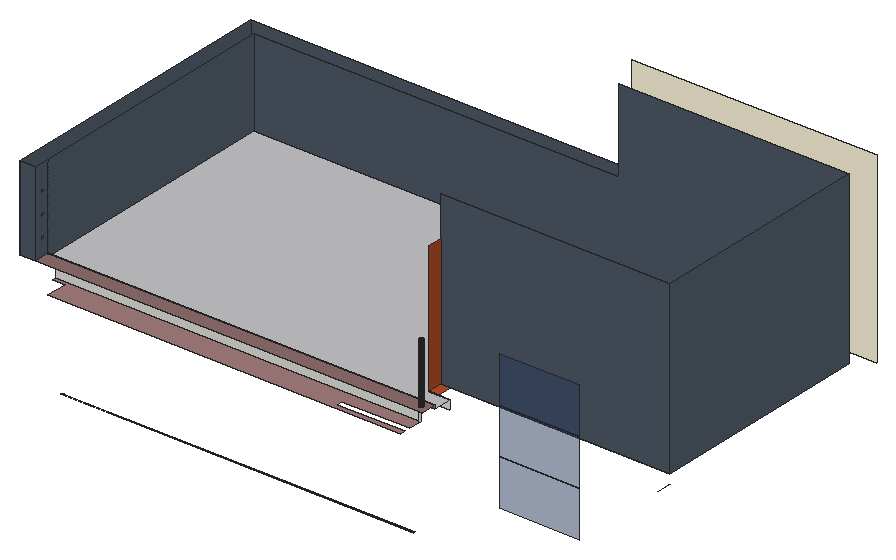
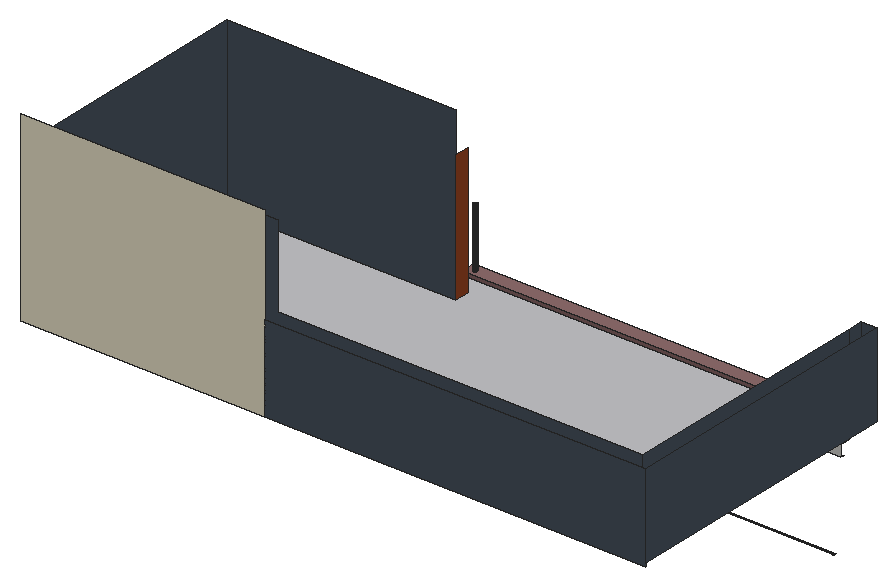
# SketchUp Ruby script. Lengths in inches.
U = 1.inch
M = Sketchup.active_model
def pt(a) = Geom::Point3d.new(a.map { |v| v * U })
def face(e, loops, mat)
  f = e.add_face(loops[0].map { |a| pt(a) })
  loops[1..].each { |l| e.add_face(l.map { |a| pt(a) }).erase! }
  f.material = f.back_material = mat if mat
  f
end
# faces: each face lists its corners as indices into pts; further lists are holes
def faces(e, pts, list, mat = nil) = list.each { |f| face(e, (f[0].is_a?(Array) ? f : [f]).map { |l| l.map { |i| pts[i] } }, mat) }
# xy, xz, yz: faces in a plane at the given z, y or x. An outline is a flat list of corners, or four numbers for a rectangle; further outlines are holes
def ring(l) = l.size == 4 ? [[l[0], l[1]], [l[2], l[1]], [l[2], l[3]], [l[0], l[3]]] : l.each_slice(2).to_a
def flat(e, list, mat, &to3) = list.each { |f| face(e, (f[0].is_a?(Array) ? f : [f]).map { |l| ring(l).map { |u, v| to3.(u, v) } }, mat) }
def xy(e, z, list, mat = nil) = flat(e, list, mat) { |x, y| [x, y, z] }
def xz(e, y, list, mat = nil) = flat(e, list, mat) { |x, z| [x, y, z] }
def yz(e, x, list, mat = nil) = flat(e, list, mat) { |y, z| [x, y, z] }
def lines(e, pts, list) = list.each { |a, b| e.add_line(pt(pts[a]), pt(pts[b])) }
# prism: a flat outline (further loops are holes) pulled along v
def prism(e, loops, v, mat = nil)
  f = face(e, loops, mat); d = Geom::Vector3d.new(v.map { |x| x * U })
  f.pushpull(f.normal.samedirection?(d) ? d.length : -d.length)
end
def box(e, o, s, mat = nil) = prism(e, [[o, [o[0] + s[0], o[1], o[2]], [o[0] + s[0], o[1] + s[1], o[2]], [o[0], o[1] + s[1], o[2]]]], [0, 0, s[2]], mat)
def at(x, y, z, deg = 0) = Geom::Transformation.translation(pt([x, y, z])) * Geom::Transformation.rotation(ORIGIN, Z_AXIS, deg.degrees)
def axes(o, x, y, z) = Geom::Transformation.new([*x, 0, *y, 0, *z, 0, *pt(o).to_a, 1])
def part(name) = M.definitions.add(name)
# library, detail: a bought-in or finely detailed component or shape, given as its bounding box
def library(name, o, s) = part(name).tap { |d| box(d.entities, o, s) }
def detail(e, o, s) = box(e.add_group.entities, o, s)
def put(e, d, t, mat = nil) = e.add_instance(d, t).tap { |i| i.material = mat if mat }
def group(e, t, mat = nil) = e.add_group.tap { |g| g.transformation = t; g.material = mat if mat }.entities
root = M.entities
M.materials.add("[0033_NavajoWhite]").color = [221, 193, 150]
M.materials.add("[0051_Cornsilk]").color = [255, 248, 220]
M.materials.add("[0111_SlateGray]").color = [79, 90, 102]
M.materials.add("[0119_RosyBrown]").color = [142, 108, 108]
M.materials.add("[0119_RosyBrown]1").color = [163, 124, 124]
M.materials.add("[0136_Charcoal]").color = [35, 35, 35]
M.materials.add("[Beadboard]").color = [181, 77, 41]
M.materials.add("[Cladding Siding Tan]").color = [162, 73, 37]
M.materials.add("[Polished Concrete New]").color = [195, 195, 198]
M.materials.add("[Translucent Glass Blue]").color = [47, 70, 112]
M.materials["[Translucent Glass Blue]"].alpha = 0.5
xy(root,2203,[[1025.375,1060.62,1025.375,1144.62,977.375,1144.62,977.375,1156.62,2393.375,1156.62,2393.375,1102.62,2129.375,1102.62,2129.375,1078.62,2393.375,1078.62,2393.375,1060.62]],"[0119_RosyBrown]1")
xy(root,2256,[[1173.81,1361.3,1167.6,1362.12,1161.81,1364.51,1156.84,1368.33,1153.02,1373.3,1150.625,1379.09,1149.81,1385.3,1150.625,1391.51,1153.02,1397.3,1156.84,1402.27,1161.81,1406.08,1167.6,1408.48,1173.81,1409.3,1180.02,1408.48,1185.81,1406.08,1190.78,1402.27,1194.59,1397.3,1196.99,1391.51,1197.81,1385.3,1196.99,1379.09,1194.59,1373.3,1190.78,1368.33,1185.81,1364.51,1180.02,1362.12],[2041.81,1361.3,2035.6,1362.12,2029.81,1364.51,2024.84,1368.33,2021.02,1373.3,2018.625,1379.09,2017.81,1385.3,2018.625,1391.51,2021.02,1397.3,2024.84,1402.27,2029.81,1406.08,2035.6,1408.48,2041.81,1409.3,2048.02,1408.48,2053.81,1406.08,2058.78,1402.27,2062.59,1397.3,2064.99,1391.51,2065.81,1385.3,2064.99,1379.09,2062.59,1373.3,2058.78,1368.33,2053.81,1364.51,2048.02,1362.12],[1173.81,1831.55,1167.6,1832.37,1161.81,1834.76,1156.84,1838.58,1153.02,1843.55,1150.625,1849.34,1149.81,1855.55,1150.625,1861.76,1153.02,1867.55,1156.84,1872.52,1161.81,1876.33,1167.6,1878.73,1173.81,1879.55,1180.02,1878.73,1185.81,1876.33,1190.78,1872.52,1194.59,1867.55,1196.99,1861.76,1197.81,1855.55,1196.99,1849.34,1194.59,1843.55,1190.78,1838.58,1185.81,1834.76,1180.02,1832.37],[2041.81,1831.55,2035.6,1832.37,2029.81,1834.76,2024.84,1838.58,2021.02,1843.55,2018.625,1849.34,2017.81,1855.55,2018.625,1861.76,2021.02,1867.55,2024.84,1872.52,2029.81,1876.33,2035.6,1878.73,2041.81,1879.55,2048.02,1878.73,2053.81,1876.33,2058.78,1872.52,2062.59,1867.55,2064.99,1861.76,2065.81,1855.55,2064.99,1849.34,2062.59,1843.55,2058.78,1838.58,2053.81,1834.76,2048.02,1832.37]])
xy(root,2256,[[[977.375,1480.62,2393.375,2116.62],[2041.81,1831.55,2048.02,1832.37,2053.81,1834.76,2058.78,1838.58,2062.59,1843.55,2064.99,1849.34,2065.81,1855.55,2064.99,1861.76,2062.59,1867.55,2058.78,1872.52,2053.81,1876.33,2048.02,1878.73,2041.81,1879.55,2035.6,1878.73,2029.81,1876.33,2024.84,1872.52,2021.02,1867.55,2018.625,1861.76,2017.81,1855.55,2018.625,1849.34,2021.02,1843.55,2024.84,1838.58,2029.81,1834.76,2035.6,1832.37],[1173.81,1831.55,1180.02,1832.37,1185.81,1834.76,1190.78,1838.58,1194.59,1843.55,1196.99,1849.34,1197.81,1855.55,1196.99,1861.76,1194.59,1867.55,1190.78,1872.52,1185.81,1876.33,1180.02,1878.73,1173.81,1879.55,1167.6,1878.73,1161.81,1876.33,1156.84,1872.52,1153.02,1867.55,1150.625,1861.76,1149.81,1855.55,1150.625,1849.34,1153.02,1843.55,1156.84,1838.58,1161.81,1834.76,1167.6,1832.37]]],"[0033_NavajoWhite]")
xy(root,2256,[[[977.375,1156.62,2393.375,1480.62],[2041.81,1361.3,2048.02,1362.12,2053.81,1364.51,2058.78,1368.33,2062.59,1373.3,2064.99,1379.09,2065.81,1385.3,2064.99,1391.51,2062.59,1397.3,2058.78,1402.27,2053.81,1406.08,2048.02,1408.48,2041.81,1409.3,2035.6,1408.48,2029.81,1406.08,2024.84,1402.27,2021.02,1397.3,2018.625,1391.51,2017.81,1385.3,2018.625,1379.09,2021.02,1373.3,2024.84,1368.33,2029.81,1364.51,2035.6,1362.12],[1173.81,1361.3,1180.02,1362.12,1185.81,1364.51,1190.78,1368.33,1194.59,1373.3,1196.99,1379.09,1197.81,1385.3,1196.99,1391.51,1194.59,1397.3,1190.78,1402.27,1185.81,1406.08,1180.02,1408.48,1173.81,1409.3,1167.6,1408.48,1161.81,1406.08,1156.84,1402.27,1153.02,1397.3,1150.625,1391.51,1149.81,1385.3,1150.625,1379.09,1153.02,1373.3,1156.84,1368.33,1161.81,1364.51,1167.6,1362.12]]],"[Beadboard]")
xy(root,2292,[[977.375,1120.62,2477.375,1120.62,2477.375,1192.62,2393.375,1192.62,2393.375,1252.62,3281.375,1252.62,3281.375,2116.62,977.375,2116.62]],"[Polished Concrete New]")
xy(root,2305.2,[[[977.375,1060.62,2477.375,1120.62],[2448.125,1082.62,2447.29,1082.66,2446.46,1082.79,2445.65,1083.01,2444.87,1083.31,2444.125,1083.6875,2443.42,1084.15,2442.77,1084.67,2442.18,1085.26,2441.65,1085.92,2441.19,1086.62,2440.81,1087.36,2440.51,1088.15,2440.3,1088.95,2440.17,1089.78,2440.125,1090.62,2440.17,1091.45,2440.3,1092.28,2440.51,1093.09,2440.81,1093.87,2441.19,1094.62,2441.65,1095.32,2442.18,1095.97,2442.77,1096.5625,2443.42,1097.09,2444.125,1097.55,2444.87,1097.93,2445.65,1098.23,2446.46,1098.44,2447.29,1098.57,2448.125,1098.62,2448.96,1098.57,2449.79,1098.44,2450.6,1098.23,2451.38,1097.93,2452.125,1097.55,2452.83,1097.09,2453.48,1096.5625,2454.07,1095.97,2454.6,1095.32,2455.05,1094.62,2455.43,1093.87,2455.73,1093.09,2455.95,1092.28,2456.08,1091.45,2456.125,1090.62,2456.08,1089.78,2455.95,1088.95,2455.73,1088.15,2455.43,1087.36,2455.05,1086.62,2454.6,1085.92,2454.07,1085.26,2453.48,1084.67,2452.83,1084.15,2452.125,1083.6875,2451.38,1083.31,2450.6,1083.01,2449.79,1082.79,2448.96,1082.66]]],"[0119_RosyBrown]")
xz(root,1060.62,[[917.375,2305.2,977.375,2630.25]],"[0111_SlateGray]")
xz(root,1120.62,[[977.375,2292,2477.375,2305.2]],"[0119_RosyBrown]")
xz(root,1156.62,[[977.375,2203,2393.375,2256]])
xz(root,1192.62,[[2393.375,2256,2477.375,2292]])
xz(root,1192.62,[[2669.375,1980,2981.375,2160],[2669.375,2160,2981.375,2340],[2669.375,2340,2981.375,2520]],"[Translucent Glass Blue]")
xz(root,1252.62,[[2393.375,2292,3281.375,2952]],"[0111_SlateGray]")
xz(root,2116.62,[[977.375,2292,3281.375,2292,3281.375,2952,2393.375,2952,2393.375,2630.25,977.375,2630.25]],"[0111_SlateGray]")
xz(root,2176.62,[[2393.375,2292,3341.375,3012]],"[0051_Cornsilk]")
xz(root,2176.62,[[917.375,2292,2393.375,2630.25]],"[0111_SlateGray]")
yz(root,917.375,[[1060.62,2305.2,2176.62,2630.25]],"[0111_SlateGray]")
yz(root,977.375,[[1120.62,2292,2116.62,2630.25],[[1060.62,2305.2,1120.62,2630.25],[1090.62,2527,1089.78,2527.04,1088.95,2527.17,1088.15,2527.39,1087.36,2527.69,1086.62,2528.07,1085.92,2528.53,1085.26,2529.05,1084.67,2529.65,1084.15,2530.3,1083.6875,2531,1083.31,2531.75,1083.01,2532.53,1082.79,2533.34,1082.66,2534.16,1082.62,2535,1082.66,2535.84,1082.79,2536.66,1083.01,2537.47,1083.31,2538.25,1083.6875,2539,1084.15,2539.7,1084.67,2540.35,1085.26,2540.95,1085.92,2541.47,1086.62,2541.93,1087.36,2542.31,1088.15,2542.61,1088.95,2542.83,1089.78,2542.96,1090.62,2543,1091.45,2542.96,1092.28,2542.83,1093.09,2542.61,1093.87,2542.31,1094.62,2541.93,1095.32,2541.47,1095.97,2540.95,1096.5625,2540.35,1097.09,2539.7,1097.55,2539,1097.93,2538.25,1098.23,2537.47,1098.44,2536.66,1098.57,2535.84,1098.62,2535,1098.57,2534.16,1098.44,2533.34,1098.23,2532.53,1097.93,2531.75,1097.55,2531,1097.09,2530.3,1096.5625,2529.65,1095.97,2529.05,1095.32,2528.53,1094.62,2528.07,1093.87,2527.69,1093.09,2527.39,1092.28,2527.17,1091.45,2527.04],[1090.62,2446,1089.78,2446.04,1088.95,2446.17,1088.15,2446.39,1087.36,2446.69,1086.62,2447.07,1085.92,2447.53,1085.26,2448.05,1084.67,2448.65,1084.15,2449.3,1083.6875,2450,1083.31,2450.75,1083.01,2451.53,1082.79,2452.34,1082.66,2453.16,1082.62,2454,1082.66,2454.84,1082.79,2455.66,1083.01,2456.47,1083.31,2457.25,1083.6875,2458,1084.15,2458.7,1084.67,2459.35,1085.26,2459.95,1085.92,2460.47,1086.62,2460.93,1087.36,2461.31,1088.15,2461.61,1088.95,2461.83,1089.78,2461.96,1090.62,2462,1091.45,2461.96,1092.28,2461.83,1093.09,2461.61,1093.87,2461.31,1094.62,2460.93,1095.32,2460.47,1095.97,2459.95,1096.5625,2459.35,1097.09,2458.7,1097.55,2458,1097.93,2457.25,1098.23,2456.47,1098.44,2455.66,1098.57,2454.84,1098.62,2454,1098.57,2453.16,1098.44,2452.34,1098.23,2451.53,1097.93,2450.75,1097.55,2450,1097.09,2449.3,1096.5625,2448.65,1095.97,2448.05,1095.32,2447.53,1094.62,2447.07,1093.87,2446.69,1093.09,2446.39,1092.28,2446.17,1091.45,2446.04],[1090.62,2365,1089.78,2365.04,1088.95,2365.17,1088.15,2365.39,1087.36,2365.69,1086.62,2366.07,1085.92,2366.53,1085.26,2367.05,1084.67,2367.65,1084.15,2368.3,1083.6875,2369,1083.31,2369.75,1083.01,2370.53,1082.79,2371.34,1082.66,2372.16,1082.62,2373,1082.66,2373.84,1082.79,2374.66,1083.01,2375.47,1083.31,2376.25,1083.6875,2377,1084.15,2377.7,1084.67,2378.35,1085.26,2378.95,1085.92,2379.47,1086.62,2379.93,1087.36,2380.31,1088.15,2380.61,1088.95,2380.83,1089.78,2380.96,1090.62,2381,1091.45,2380.96,1092.28,2380.83,1093.09,2380.61,1093.87,2380.31,1094.62,2379.93,1095.32,2379.47,1095.97,2378.95,1096.5625,2378.35,1097.09,2377.7,1097.55,2377,1097.93,2376.25,1098.23,2375.47,1098.44,2374.66,1098.57,2373.84,1098.62,2373,1098.57,2372.16,1098.44,2371.34,1098.23,2370.53,1097.93,2369.75,1097.55,2369,1097.09,2368.3,1096.5625,2367.65,1095.97,2367.05,1095.32,2366.53,1094.62,2366.07,1093.87,2365.69,1093.09,2365.39,1092.28,2365.17,1091.45,2365.04]]],"[0111_SlateGray]")
yz(root,2393.375,[[1144.62,2203,1156.62,2256]])
yz(root,2393.375,[[1192.62,2292,1252.62,2796]],"[Cladding Siding Tan]")
yz(root,3281.375,[[1252.62,2292,2116.62,2952]],"[0111_SlateGray]")
p = [[1025.375,1122.58,1833.86],[1025.375,1121.62,1833.46],[2393.375,1121.62,1833.46],[2393.375,1122.58,1833.86],[1025.375,1125.62,1833.46],[1025.375,1124.65,1833.86],
  [2393.375,1124.65,1833.86],[2393.375,1125.62,1833.46],[1025.375,1123.62,1834],[2393.375,1123.62,1834],[2447.29,1082.66,2372.16],[2447.29,1082.66,2305.2],
  [2448.125,1082.62,2305.2],[2448.125,1082.62,2373],[2448.125,1082.62,2454],[2448.125,1082.62,2535],[2448.125,1082.62,2536.5],[2447.29,1082.66,2536.5],
  [2447.29,1082.66,2535.84],[2447.29,1082.66,2534.16],[2447.29,1082.66,2454.84],[2447.29,1082.66,2453.16],[2447.29,1082.66,2373.84],[2448.96,1082.66,2305.2],
  [2448.96,1082.66,2372.16],[2448.96,1082.66,2373.84],[2448.96,1082.66,2453.16],[2448.96,1082.66,2454.84],[2448.96,1082.66,2534.16],[2448.96,1082.66,2535.84],
  [2448.96,1082.66,2536.5],[2446.46,1082.79,2371.34],[2446.46,1082.79,2305.2],[2446.46,1082.79,2536.5],[2446.46,1082.79,2533.34],[2446.46,1082.79,2455.66],
  [2446.46,1082.79,2452.34],[2446.46,1082.79,2374.66],[2449.79,1082.79,2305.2],[2449.79,1082.79,2371.34],[2449.79,1082.79,2374.66],[2449.79,1082.79,2452.34],
  [2449.79,1082.79,2455.66],[2449.79,1082.79,2533.34],[2449.79,1082.79,2536.5],[2445.65,1083.01,2370.53],[2445.65,1083.01,2305.2],[2445.65,1083.01,2536.5],
  [2445.65,1083.01,2532.53],[2445.65,1083.01,2456.47],[2445.65,1083.01,2451.53],[2445.65,1083.01,2375.47],[2450.6,1083.01,2305.2],[2450.6,1083.01,2370.53],
  [2450.6,1083.01,2375.47],[2450.6,1083.01,2451.53],[2450.6,1083.01,2456.47],[2450.6,1083.01,2532.53],[2450.6,1083.01,2536.5],[2444.87,1083.31,2369.75],
  [2444.87,1083.31,2305.2],[2444.87,1083.31,2536.5],[2444.87,1083.31,2531.75],[2444.87,1083.31,2457.25],[2444.87,1083.31,2450.75],[2444.87,1083.31,2376.25],
  [2451.38,1083.31,2305.2],[2451.38,1083.31,2369.75],[2451.38,1083.31,2376.25],[2451.38,1083.31,2450.75],[2451.38,1083.31,2457.25],[2451.38,1083.31,2531.75],
  [2451.38,1083.31,2536.5],[2444.125,1083.6875,2369],[2444.125,1083.6875,2305.2],[2444.125,1083.6875,2536.5],[2444.125,1083.6875,2531],[2444.125,1083.6875,2458],
  [2444.125,1083.6875,2450],[2444.125,1083.6875,2377],[2452.125,1083.6875,2305.2],[2452.125,1083.6875,2369],[2452.125,1083.6875,2377],[2452.125,1083.6875,2450],
  [2452.125,1083.6875,2458],[2452.125,1083.6875,2531],[2452.125,1083.6875,2536.5],[2443.42,1084.15,2368.3],[2443.42,1084.15,2305.2],[2443.42,1084.15,2536.5],
  [2443.42,1084.15,2530.3],[2443.42,1084.15,2458.7],[2443.42,1084.15,2449.3],[2443.42,1084.15,2377.7],[2452.83,1084.15,2305.2],[2452.83,1084.15,2368.3],
  [2452.83,1084.15,2377.7],[2452.83,1084.15,2449.3],[2452.83,1084.15,2458.7],[2452.83,1084.15,2530.3],[2452.83,1084.15,2536.5],[2442.77,1084.67,2367.65],
  [2442.77,1084.67,2305.2],[2442.77,1084.67,2536.5],[2442.77,1084.67,2529.65],[2442.77,1084.67,2459.35],[2442.77,1084.67,2448.65],[2442.77,1084.67,2378.35],
  [2453.48,1084.67,2305.2],[2453.48,1084.67,2367.65],[2453.48,1084.67,2378.35],[2453.48,1084.67,2448.65],[2453.48,1084.67,2459.35],[2453.48,1084.67,2529.65],
  [2453.48,1084.67,2536.5],[2442.18,1085.26,2367.05],[2442.18,1085.26,2305.2],[2442.18,1085.26,2536.5],[2442.18,1085.26,2529.05],[2442.18,1085.26,2459.95],
  [2442.18,1085.26,2448.05],[2442.18,1085.26,2378.95],[2454.07,1085.26,2305.2],[2454.07,1085.26,2367.65],[2454.07,1085.26,2378.35],[2454.07,1085.26,2448.65],
  [2454.07,1085.26,2459.35],[2454.07,1085.26,2529.65],[2454.07,1085.26,2536.5],[2441.65,1085.92,2366.53],[2441.65,1085.92,2305.2],[2441.65,1085.92,2536.5],
  [2441.65,1085.92,2528.53],[2441.65,1085.92,2460.47],[2441.65,1085.92,2447.53],[2441.65,1085.92,2379.47],[2454.6,1085.92,2305.2],[2454.6,1085.92,2368.3],
  [2454.6,1085.92,2377.7],[2454.6,1085.92,2449.3],[2454.6,1085.92,2458.7],[2454.6,1085.92,2530.3],[2454.6,1085.92,2536.5],[2441.19,1086.62,2366.07],
  [2441.19,1086.62,2305.2],[2441.19,1086.62,2536.5],[2441.19,1086.62,2528.07],[2441.19,1086.62,2460.93],[2441.19,1086.62,2447.07],[2441.19,1086.62,2379.93],
  [2455.05,1086.62,2305.2],[2455.05,1086.62,2369],[2455.05,1086.62,2377],[2455.05,1086.62,2450],[2455.05,1086.62,2458],[2455.05,1086.62,2531],
  [2455.05,1086.62,2536.5],[2440.81,1087.36,2365.69],[2440.81,1087.36,2305.2],[2440.81,1087.36,2536.5],[2440.81,1087.36,2527.69],[2440.81,1087.36,2461.31],
  [2440.81,1087.36,2446.69],[2440.81,1087.36,2380.31],[2455.43,1087.36,2305.2],[2455.43,1087.36,2369.75],[2455.43,1087.36,2376.25],[2455.43,1087.36,2450.75],
  [2455.43,1087.36,2457.25],[2455.43,1087.36,2531.75],[2455.43,1087.36,2536.5],[2440.51,1088.15,2365.39],[2440.51,1088.15,2305.2],[2440.51,1088.15,2536.5],
  [2440.51,1088.15,2527.39],[2440.51,1088.15,2461.61],[2440.51,1088.15,2446.39],[2440.51,1088.15,2380.61],[2455.73,1088.15,2305.2],[2455.73,1088.15,2370.53],
  [2455.73,1088.15,2375.47],[2455.73,1088.15,2451.53],[2455.73,1088.15,2456.47],[2455.73,1088.15,2532.53],[2455.73,1088.15,2536.5],[2440.3,1088.95,2365.17],
  [2440.3,1088.95,2305.2],[2440.3,1088.95,2536.5],[2440.3,1088.95,2527.17],[2440.3,1088.95,2461.83],[2440.3,1088.95,2446.17],[2440.3,1088.95,2380.83],
  [2455.95,1088.95,2305.2],[2455.95,1088.95,2371.34],[2455.95,1088.95,2374.66],[2455.95,1088.95,2452.34],[2455.95,1088.95,2455.66],[2455.95,1088.95,2533.34],
  [2455.95,1088.95,2536.5],[2440.17,1089.78,2365.04],[2440.17,1089.78,2305.2],[2440.17,1089.78,2536.5],[2440.17,1089.78,2527.04],[2440.17,1089.78,2461.96],
  [2440.17,1089.78,2446.04],[2440.17,1089.78,2380.96],[2456.08,1089.78,2305.2],[2456.08,1089.78,2372.16],[2456.08,1089.78,2373.84],[2456.08,1089.78,2453.16],
  [2456.08,1089.78,2454.84],[2456.08,1089.78,2534.16],[2456.08,1089.78,2535.84],[2456.08,1089.78,2536.5],[2440.125,1090.62,2365],[2440.125,1090.62,2305.2],
  [2440.125,1090.62,2536.5],[2440.125,1090.62,2535],[2440.125,1090.62,2527],[2440.125,1090.62,2462],[2440.125,1090.62,2454],[2440.125,1090.62,2446],
  [2440.125,1090.62,2381],[2440.125,1090.62,2373],[2456.125,1090.62,2305.2],[2456.125,1090.62,2373],[2456.125,1090.62,2454],[2456.125,1090.62,2535],
  [2456.125,1090.62,2536.5],[2440.17,1091.45,2365.04],[2440.17,1091.45,2305.2],[2440.17,1091.45,2536.5],[2440.17,1091.45,2527.04],[2440.17,1091.45,2461.96],
  [2440.17,1091.45,2446.04],[2440.17,1091.45,2380.96],[2456.08,1091.45,2305.2],[2456.08,1091.45,2372.16],[2456.08,1091.45,2373.84],[2456.08,1091.45,2453.16],
  [2456.08,1091.45,2454.84],[2456.08,1091.45,2534.16],[2456.08,1091.45,2535.84],[2456.08,1091.45,2536.5],[2440.3,1092.28,2365.17],[2440.3,1092.28,2305.2],
  [2440.3,1092.28,2536.5],[2440.3,1092.28,2527.17],[2440.3,1092.28,2461.83],[2440.3,1092.28,2446.17],[2440.3,1092.28,2380.83],[2455.95,1092.28,2305.2],
  [2455.95,1092.28,2371.34],[2455.95,1092.28,2374.66],[2455.95,1092.28,2452.34],[2455.95,1092.28,2455.66],[2455.95,1092.28,2533.34],[2455.95,1092.28,2536.5],
  [2440.51,1093.09,2365.39],[2440.51,1093.09,2305.2],[2440.51,1093.09,2536.5],[2440.51,1093.09,2527.39],[2440.51,1093.09,2461.61],[2440.51,1093.09,2446.39],
  [2440.51,1093.09,2380.61],[2455.73,1093.09,2305.2],[2455.73,1093.09,2370.53],[2455.73,1093.09,2375.47],[2455.73,1093.09,2451.53],[2455.73,1093.09,2456.47],
  [2455.73,1093.09,2532.53],[2455.73,1093.09,2536.5],[2440.81,1093.87,2365.69],[2440.81,1093.87,2305.2],[2440.81,1093.87,2536.5],[2440.81,1093.87,2527.69],
  [2440.81,1093.87,2461.31],[2440.81,1093.87,2446.69],[2440.81,1093.87,2380.31],[2455.43,1093.87,2305.2],[2455.43,1093.87,2369.75],[2455.43,1093.87,2376.25],
  [2455.43,1093.87,2450.75],[2455.43,1093.87,2457.25],[2455.43,1093.87,2531.75],[2455.43,1093.87,2536.5],[2441.19,1094.62,2366.07],[2441.19,1094.62,2305.2],
  [2441.19,1094.62,2536.5],[2441.19,1094.62,2528.07],[2441.19,1094.62,2460.93],[2441.19,1094.62,2447.07],[2441.19,1094.62,2379.93],[2455.05,1094.62,2305.2],
  [2455.05,1094.62,2369],[2455.05,1094.62,2377],[2455.05,1094.62,2450],[2455.05,1094.62,2458],[2455.05,1094.62,2531],[2455.05,1094.62,2536.5],
  [2441.65,1095.32,2366.53],[2441.65,1095.32,2305.2],[2441.65,1095.32,2536.5],[2441.65,1095.32,2528.53],[2441.65,1095.32,2460.47],[2441.65,1095.32,2447.53],
  [2441.65,1095.32,2379.47],[2454.6,1095.32,2305.2],[2454.6,1095.32,2368.3],[2454.6,1095.32,2377.7],[2454.6,1095.32,2449.3],[2454.6,1095.32,2458.7],
  [2454.6,1095.32,2530.3],[2454.6,1095.32,2536.5],[2442.18,1095.97,2367.05],[2442.18,1095.97,2305.2],[2442.18,1095.97,2536.5],[2442.18,1095.97,2529.05],
  [2442.18,1095.97,2459.95],[2442.18,1095.97,2448.05],[2442.18,1095.97,2378.95],[2454.07,1095.97,2305.2],[2454.07,1095.97,2367.65],[2454.07,1095.97,2378.35],
  [2454.07,1095.97,2448.65],[2454.07,1095.97,2459.35],[2454.07,1095.97,2529.65],[2454.07,1095.97,2536.5],[2442.77,1096.5625,2367.05],[2442.77,1096.5625,2305.2],
  [2442.77,1096.5625,2536.5],[2442.77,1096.5625,2529.05],[2442.77,1096.5625,2459.95],[2442.77,1096.5625,2448.05],[2442.77,1096.5625,2378.95],[2453.48,1096.5625,2305.2],
  [2453.48,1096.5625,2367.05],[2453.48,1096.5625,2378.95],[2453.48,1096.5625,2448.05],[2453.48,1096.5625,2459.95],[2453.48,1096.5625,2529.05],[2453.48,1096.5625,2536.5],
  [2443.42,1097.09,2366.53],[2443.42,1097.09,2305.2],[2443.42,1097.09,2536.5],[2443.42,1097.09,2528.53],[2443.42,1097.09,2460.47],[2443.42,1097.09,2447.53],
  [2443.42,1097.09,2379.47],[2452.83,1097.09,2305.2],[2452.83,1097.09,2366.53],[2452.83,1097.09,2379.47],[2452.83,1097.09,2447.53],[2452.83,1097.09,2460.47],
  [2452.83,1097.09,2528.53],[2452.83,1097.09,2536.5],[2444.125,1097.55,2366.07],[2444.125,1097.55,2305.2],[2444.125,1097.55,2536.5],[2444.125,1097.55,2528.07],
  [2444.125,1097.55,2460.93],[2444.125,1097.55,2447.07],[2444.125,1097.55,2379.93],[2452.125,1097.55,2305.2],[2452.125,1097.55,2366.07],[2452.125,1097.55,2379.93],
  [2452.125,1097.55,2447.07],[2452.125,1097.55,2460.93],[2452.125,1097.55,2528.07],[2452.125,1097.55,2536.5],[2444.87,1097.93,2365.69],[2444.87,1097.93,2305.2],
  [2444.87,1097.93,2536.5],[2444.87,1097.93,2527.69],[2444.87,1097.93,2461.31],[2444.87,1097.93,2446.69],[2444.87,1097.93,2380.31],[2451.38,1097.93,2305.2],
  [2451.38,1097.93,2365.69],[2451.38,1097.93,2380.31],[2451.38,1097.93,2446.69],[2451.38,1097.93,2461.31],[2451.38,1097.93,2527.69],[2451.38,1097.93,2536.5],
  [2445.65,1098.23,2365.39],[2445.65,1098.23,2305.2],[2445.65,1098.23,2536.5],[2445.65,1098.23,2527.39],[2445.65,1098.23,2461.61],[2445.65,1098.23,2446.39],
  [2445.65,1098.23,2380.61],[2450.6,1098.23,2305.2],[2450.6,1098.23,2365.39],[2450.6,1098.23,2380.61],[2450.6,1098.23,2446.39],[2450.6,1098.23,2461.61],
  [2450.6,1098.23,2527.39],[2450.6,1098.23,2536.5],[2446.46,1098.44,2365.17],[2446.46,1098.44,2305.2],[2446.46,1098.44,2536.5],[2446.46,1098.44,2527.17],
  [2446.46,1098.44,2461.83],[2446.46,1098.44,2446.17],[2446.46,1098.44,2380.83],[2449.79,1098.44,2305.2],[2449.79,1098.44,2365.17],[2449.79,1098.44,2380.83],
  [2449.79,1098.44,2446.17],[2449.79,1098.44,2461.83],[2449.79,1098.44,2527.17],[2449.79,1098.44,2536.5],[2447.29,1098.57,2365.04],[2447.29,1098.57,2305.2],
  [2447.29,1098.57,2536.5],[2447.29,1098.57,2527.04],[2447.29,1098.57,2461.96],[2447.29,1098.57,2446.04],[2447.29,1098.57,2380.96],[2448.96,1098.57,2305.2],
  [2448.96,1098.57,2365.04],[2448.96,1098.57,2380.96],[2448.96,1098.57,2446.04],[2448.96,1098.57,2461.96],[2448.96,1098.57,2527.04],[2448.96,1098.57,2536.5],
  [2448.125,1098.62,2365],[2448.125,1098.62,2305.2],[2448.125,1098.62,2536.5],[2448.125,1098.62,2535],[2448.125,1098.62,2527],[2448.125,1098.62,2462],
  [2448.125,1098.62,2454],[2448.125,1098.62,2446],[2448.125,1098.62,2381],[2448.125,1098.62,2373],[3281.375,1252.62,2256],[3281.375,1192.62,2256],
  [2393.375,2176.62,2292],[2393.375,2116.62,2292],[2448.125,1090.62,2292],[2448.125,1090.62,2365]]
faces(root,p,[[0,1,2,3],[4,5,6,7],[8,0,3,9],[5,8,9,6],[10,11,12,13,14,15,16,17,18,19,20,21,22],[13,12,23,24,25,26,27,28,29,30,16,15,14],[31,32,11,10,22,21,20,19,18,17,33,34,35,36,37],[24,23,38,39,40,41,42,43,44,30,29,28,27,26,25],
  [45,46,32,31,37,36,35,34,33,47,48,49,50,51],[39,38,52,53,54,55,56,57,58,44,43,42,41,40],[59,60,46,45,51,50,49,48,47,61,62,63,64,65],[53,52,66,67,68,69,70,71,72,58,57,56,55,54],[73,74,60,59,65,64,63,62,61,75,76,77,78,79],[67,66,80,81,82,83,84,85,86,72,71,70,69,68],[87,88,74,73,79,78,77,76,75,89,90,91,92,93],[81,80,94,95,96,97,98,99,100,86,85,84,83,82],
  [101,102,88,87,93,92,91,90,89,103,104,105,106,107],[95,94,108,109,110,111,112,113,114,100,99,98,97,96],[115,116,102,101,107,106,105,104,103,117,118,119,120,121],[109,108,122,123,124,125,126,127,128,114,113,112,111,110],[129,130,116,115,121,120,119,118,117,131,132,133,134,135],[123,122,136,137,138,139,140,141,142,128,127,126,125,124],[143,144,130,129,135,134,133,132,131,145,146,147,148,149],[137,136,150,151,152,153,154,155,156,142,141,140,139,138],
  [157,158,144,143,149,148,147,146,145,159,160,161,162,163],[151,150,164,165,166,167,168,169,170,156,155,154,153,152],[171,172,158,157,163,162,161,160,159,173,174,175,176,177],[165,164,178,179,180,181,182,183,184,170,169,168,167,166],[185,186,172,171,177,176,175,174,173,187,188,189,190,191],[179,178,192,193,194,195,196,197,198,184,183,182,181,180],[199,200,186,185,191,190,189,188,187,201,202,203,204,205],[193,192,206,207,208,209,210,211,212,213,198,197,196,195,194],
  [214,215,200,199,205,204,203,202,201,216,217,218,219,220,221,222,223],[207,206,224,225,226,227,228,213,212,211,210,209,208],[229,230,215,214,223,222,221,220,219,218,217,216,231,232,233,234,235],[225,224,236,237,238,239,240,241,242,243,228,227,226],[244,245,230,229,235,234,233,232,231,246,247,248,249,250],[237,236,251,252,253,254,255,256,257,243,242,241,240,239,238],[258,259,245,244,250,249,248,247,246,260,261,262,263,264],[252,251,265,266,267,268,269,270,271,257,256,255,254,253],
  [272,273,259,258,264,263,262,261,260,274,275,276,277,278],[266,265,279,280,281,282,283,284,285,271,270,269,268,267],[286,287,273,272,278,277,276,275,274,288,289,290,291,292],[280,279,293,294,295,296,297,298,299,285,284,283,282,281],[300,301,287,286,292,291,290,289,288,302,303,304,305,306],[294,293,307,308,309,310,311,312,313,299,298,297,296,295],[314,315,301,300,306,305,304,303,302,316,317,318,319,320],[308,307,321,322,323,324,325,326,327,313,312,311,310,309],
  [328,329,315,314,320,319,318,317,316,330,331,332,333,334],[322,321,335,336,337,338,339,340,341,327,326,325,324,323],[342,343,329,328,334,333,332,331,330,344,345,346,347,348],[336,335,349,350,351,352,353,354,355,341,340,339,338,337],[356,357,343,342,348,347,346,345,344,358,359,360,361,362],[350,349,363,364,365,366,367,368,369,355,354,353,352,351],[370,371,357,356,362,361,360,359,358,372,373,374,375,376],[364,363,377,378,379,380,381,382,383,369,368,367,366,365],
  [384,385,371,370,376,375,374,373,372,386,387,388,389,390],[378,377,391,392,393,394,395,396,397,383,382,381,380,379],[398,399,385,384,390,389,388,387,386,400,401,402,403,404],[392,391,405,406,407,408,409,410,411,397,396,395,394,393],[412,413,399,398,404,403,402,401,400,414,415,416,417,418],[406,405,419,420,421,422,423,424,425,411,410,409,408,407],[426,427,413,412,418,417,416,415,414,428,429,430,431,432,433,434,435],[420,419,427,426,435,434,433,432,431,430,429,428,425,424,423,422,421]],"[0136_Charcoal]")
lines(root,p,[[436,437],[438,439],[440,441]])
